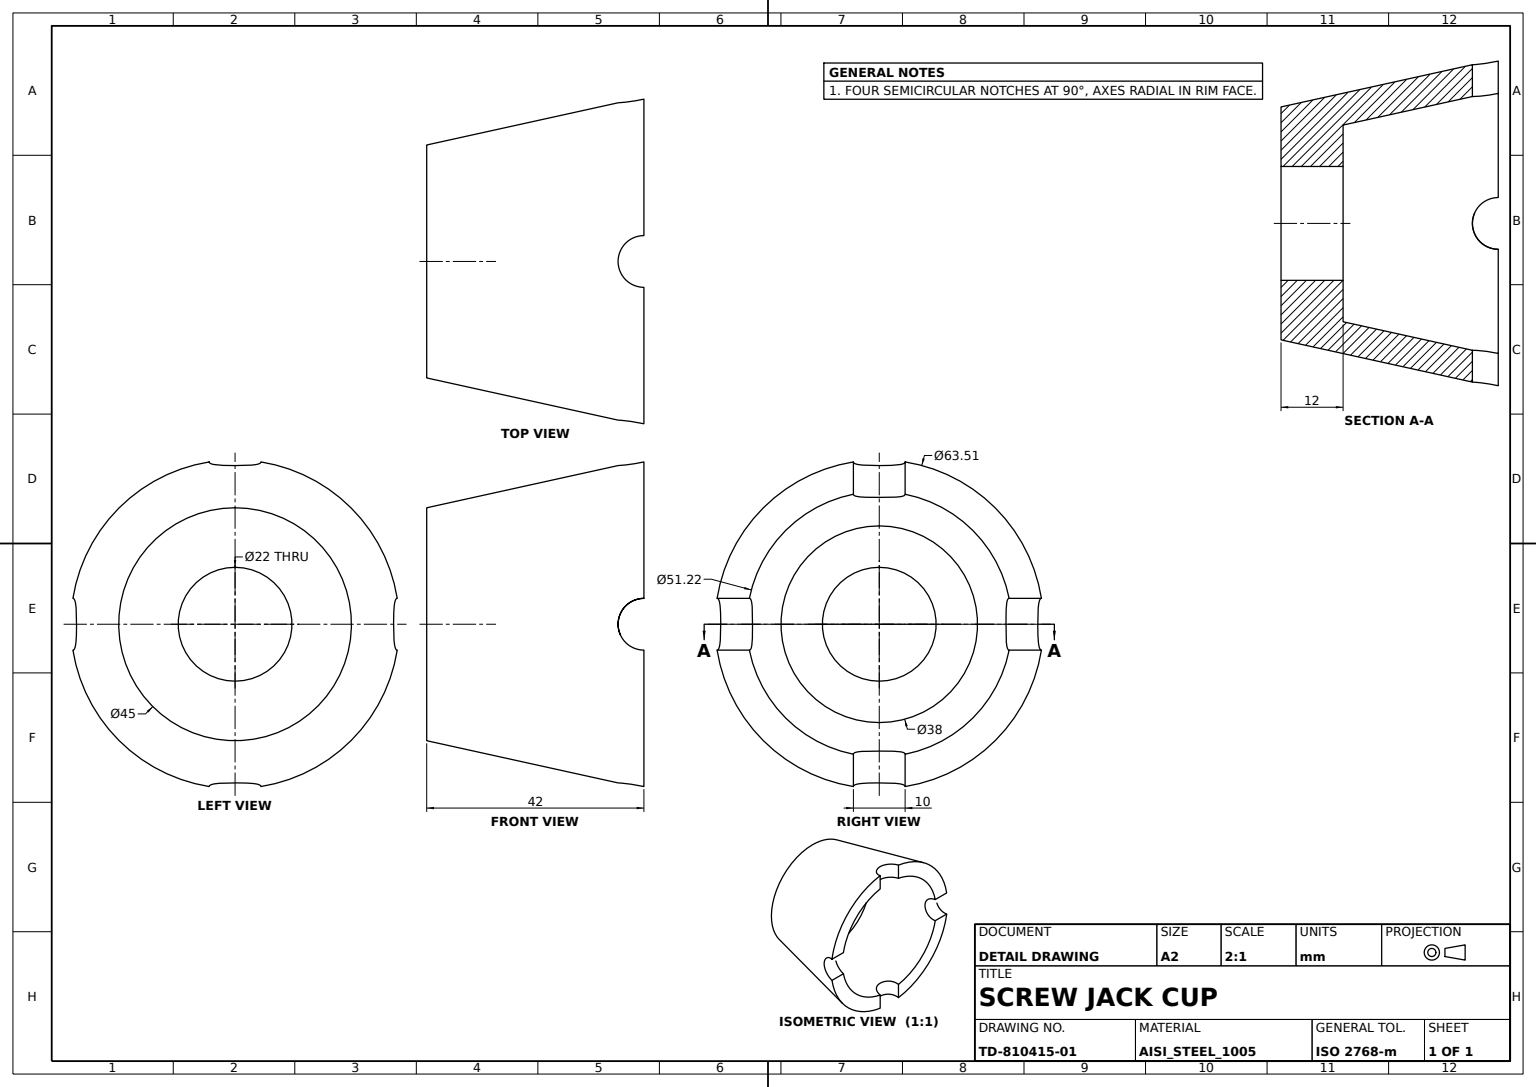
ISO-10303-21;
HEADER;
FILE_DESCRIPTION((''),'2;1');
FILE_NAME('','',(''),(''),'','','');
FILE_SCHEMA(('AUTOMOTIVE_DESIGN'));
ENDSEC;
DATA;
#1=APPLICATION_CONTEXT('');
#2=PRODUCT_CONTEXT('',#1,'mechanical');
#3=PRODUCT('','','',(#2));
#4=PRODUCT_DEFINITION_FORMATION('','',#3);
#5=PRODUCT_DEFINITION_CONTEXT('',#1,'design');
#6=PRODUCT_DEFINITION('','',#4,#5);
#7=PRODUCT_DEFINITION_SHAPE('','',#6);
#8=(LENGTH_UNIT()NAMED_UNIT(*)SI_UNIT(.MILLI.,.METRE.));
#9=(NAMED_UNIT(*)PLANE_ANGLE_UNIT()SI_UNIT($,.RADIAN.));
#10=(NAMED_UNIT(*)SI_UNIT($,.STERADIAN.)SOLID_ANGLE_UNIT());
#11=UNCERTAINTY_MEASURE_WITH_UNIT(LENGTH_MEASURE(0.005),#8,'distance_accuracy_value','');
#12=(GEOMETRIC_REPRESENTATION_CONTEXT(3)GLOBAL_UNCERTAINTY_ASSIGNED_CONTEXT((#11))GLOBAL_UNIT_ASSIGNED_CONTEXT((#8,#9,#10))REPRESENTATION_CONTEXT('',''));
#13=CARTESIAN_POINT('',(-42.,-25.116923,5.));
#14=VERTEX_POINT('',#13);
#15=CARTESIAN_POINT('',(-42.,-25.116923,-5.));
#16=VERTEX_POINT('',#15);
#17=CARTESIAN_POINT('',(-41.352204,-24.971396,5.));
#18=CARTESIAN_POINT('',(-40.063797,-24.73353,4.748155));
#19=CARTESIAN_POINT('',(-37.824304,-24.500184,3.278245));
#20=CARTESIAN_POINT('',(-36.450174,-24.515156,0.008023));
#21=CARTESIAN_POINT('',(-38.100183,-24.490988,-3.940384));
#22=CARTESIAN_POINT('',(-40.704221,-24.825828,-5.));
#23=B_SPLINE_CURVE_WITH_KNOTS('',3,(#13,#17,#18,#19,#20,#21,#22,#15),.UNSPECIFIED.,.F.,.F.,(4,1,1,1,1,4),(0.000000202,0.001964487,0.003928772,0.007857341,0.01178591,0.01571448),.UNSPECIFIED.);
#24=EDGE_CURVE('',#14,#16,#23,.T.);
#25=ORIENTED_EDGE('',*,*,#24,.T.);
#26=CARTESIAN_POINT('',(-42.,-31.357538,-5.));
#27=VERTEX_POINT('',#26);
#28=CARTESIAN_POINT('',(-42.,-40.,-5.));
#29=DIRECTION('',(0.,1.,0.));
#30=VECTOR('',#29,1000.);
#31=LINE('',#28,#30);
#32=EDGE_CURVE('',#27,#16,#31,.T.);
#33=ORIENTED_EDGE('',*,*,#32,.F.);
#34=CARTESIAN_POINT('',(-42.,-31.357538,5.));
#35=VERTEX_POINT('',#34);
#36=CARTESIAN_POINT('',(-41.351427,-31.212836,-5.));
#37=CARTESIAN_POINT('',(-40.064058,-30.966956,-4.747835));
#38=CARTESIAN_POINT('',(-37.826606,-30.682429,-3.280684));
#39=CARTESIAN_POINT('',(-36.448665,-30.633085,-0.008));
#40=CARTESIAN_POINT('',(-38.103157,-30.687587,3.942255));
#41=CARTESIAN_POINT('',(-40.702699,-31.068099,5.));
#42=B_SPLINE_CURVE_WITH_KNOTS('',3,(#26,#36,#37,#38,#39,#40,#41,#34),.UNSPECIFIED.,.F.,.F.,(4,1,1,1,1,4),(0.000000202,0.001966139,0.003932077,0.007863951,0.011795825,0.0157277),.UNSPECIFIED.);
#43=EDGE_CURVE('',#27,#35,#42,.T.);
#44=ORIENTED_EDGE('',*,*,#43,.T.);
#45=CARTESIAN_POINT('',(-42.,-40.,5.));
#46=LINE('',#45,#30);
#47=EDGE_CURVE('',#14,#35,#46,.F.);
#48=ORIENTED_EDGE('',*,*,#47,.F.);
#49=EDGE_LOOP('',(#25,#33,#44,#48));
#50=FACE_BOUND('',#49,.T.);
#51=CARTESIAN_POINT('',(-42.,-40.,0.));
#52=DIRECTION('',(0.,0.,1.));
#53=AXIS2_PLACEMENT_3D('',#51,#29,#52);
#54=CYLINDRICAL_SURFACE('',#53,5.);
#55=ADVANCED_FACE('',(#50),#54,.F.);
#56=CARTESIAN_POINT('',(-42.,5.,-31.357538));
#57=VERTEX_POINT('',#56);
#58=CARTESIAN_POINT('',(-42.,5.,-25.116923));
#59=VERTEX_POINT('',#58);
#60=CARTESIAN_POINT('',(-42.,5.,-40.));
#61=VECTOR('',#52,1000.);
#62=LINE('',#60,#61);
#63=EDGE_CURVE('',#57,#59,#62,.T.);
#64=ORIENTED_EDGE('',*,*,#63,.T.);
#65=CARTESIAN_POINT('',(-42.,25.116923,-5.));
#66=VERTEX_POINT('',#65);
#67=CARTESIAN_POINT('',(-42.,0.,0.));
#68=DIRECTION('',(-1.,0.,0.));
#69=AXIS2_PLACEMENT_3D('',#67,#68,#52);
#70=CIRCLE('',#69,25.60976);
#71=EDGE_CURVE('',#66,#59,#70,.T.);
#72=ORIENTED_EDGE('',*,*,#71,.F.);
#73=CARTESIAN_POINT('',(-42.,31.357538,-5.));
#74=VERTEX_POINT('',#73);
#75=CARTESIAN_POINT('',(-42.,40.,-5.));
#76=DIRECTION('',(0.,-1.,0.));
#77=VECTOR('',#76,1000.);
#78=LINE('',#75,#77);
#79=EDGE_CURVE('',#66,#74,#78,.F.);
#80=ORIENTED_EDGE('',*,*,#79,.T.);
#81=CIRCLE('',#69,31.753664);
#82=EDGE_CURVE('',#74,#57,#81,.T.);
#83=ORIENTED_EDGE('',*,*,#82,.T.);
#84=EDGE_LOOP('',(#64,#72,#80,#83));
#85=FACE_BOUND('',#84,.T.);
#86=CARTESIAN_POINT('',(-42.,31.753664,0.));
#87=DIRECTION('',(1.,0.,0.));
#88=DIRECTION('',(0.,0.,-1.));
#89=AXIS2_PLACEMENT_3D('',#86,#87,#88);
#90=PLANE('',#89);
#91=ADVANCED_FACE('',(#85),#90,.F.);
#92=CARTESIAN_POINT('',(0.,0.,22.5));
#93=VERTEX_POINT('',#92);
#94=CARTESIAN_POINT('',(0.,0.,0.));
#95=AXIS2_PLACEMENT_3D('',#94,#68,#52);
#96=CIRCLE('',#95,22.5);
#97=EDGE_CURVE('',#93,#93,#96,.T.);
#98=ORIENTED_EDGE('',*,*,#97,.T.);
#99=EDGE_LOOP('',(#98));
#100=FACE_BOUND('',#99,.T.);
#101=ORIENTED_EDGE('',*,*,#43,.F.);
#102=CARTESIAN_POINT('',(-42.,-5.,-31.357538));
#103=VERTEX_POINT('',#102);
#104=EDGE_CURVE('',#103,#27,#81,.T.);
#105=ORIENTED_EDGE('',*,*,#104,.F.);
#106=CARTESIAN_POINT('',(-41.351427,5.,-31.212836));
#107=CARTESIAN_POINT('',(-40.064058,4.747835,-30.966956));
#108=CARTESIAN_POINT('',(-37.826606,3.280684,-30.682429));
#109=CARTESIAN_POINT('',(-36.448665,0.008,-30.633085));
#110=CARTESIAN_POINT('',(-38.103157,-3.942255,-30.687587));
#111=CARTESIAN_POINT('',(-40.702699,-5.,-31.068099));
#112=B_SPLINE_CURVE_WITH_KNOTS('',3,(#56,#106,#107,#108,#109,#110,#111,#102),.UNSPECIFIED.,.F.,.F.,(4,1,1,1,1,4),(0.000000202,0.001966139,0.003932077,0.007863951,0.011795825,0.0157277),.UNSPECIFIED.);
#113=EDGE_CURVE('',#57,#103,#112,.T.);
#114=ORIENTED_EDGE('',*,*,#113,.F.);
#115=ORIENTED_EDGE('',*,*,#82,.F.);
#116=CARTESIAN_POINT('',(-42.,31.357538,5.));
#117=VERTEX_POINT('',#116);
#118=CARTESIAN_POINT('',(-41.351427,31.212836,5.));
#119=CARTESIAN_POINT('',(-40.064058,30.966956,4.747835));
#120=CARTESIAN_POINT('',(-37.826606,30.682429,3.280684));
#121=CARTESIAN_POINT('',(-36.448665,30.633085,0.008));
#122=CARTESIAN_POINT('',(-38.103157,30.687587,-3.942255));
#123=CARTESIAN_POINT('',(-40.702699,31.068099,-5.));
#124=B_SPLINE_CURVE_WITH_KNOTS('',3,(#116,#118,#119,#120,#121,#122,#123,#73),.UNSPECIFIED.,.F.,.F.,(4,1,1,1,1,4),(0.000000202,0.001966139,0.003932077,0.007863951,0.011795825,0.0157277),.UNSPECIFIED.);
#125=EDGE_CURVE('',#117,#74,#124,.T.);
#126=ORIENTED_EDGE('',*,*,#125,.F.);
#127=CARTESIAN_POINT('',(-42.,5.,31.357538));
#128=VERTEX_POINT('',#127);
#129=EDGE_CURVE('',#128,#117,#81,.T.);
#130=ORIENTED_EDGE('',*,*,#129,.F.);
#131=CARTESIAN_POINT('',(-42.,-5.,31.357538));
#132=VERTEX_POINT('',#131);
#133=CARTESIAN_POINT('',(-41.351427,-5.,31.212836));
#134=CARTESIAN_POINT('',(-40.064058,-4.747835,30.966956));
#135=CARTESIAN_POINT('',(-37.826606,-3.280684,30.682429));
#136=CARTESIAN_POINT('',(-36.448665,-0.008,30.633085));
#137=CARTESIAN_POINT('',(-38.103157,3.942255,30.687587));
#138=CARTESIAN_POINT('',(-40.702699,5.,31.068099));
#139=B_SPLINE_CURVE_WITH_KNOTS('',3,(#131,#133,#134,#135,#136,#137,#138,#127),.UNSPECIFIED.,.F.,.F.,(4,1,1,1,1,4),(0.000000202,0.001966139,0.003932077,0.007863951,0.011795825,0.0157277),.UNSPECIFIED.);
#140=EDGE_CURVE('',#132,#128,#139,.T.);
#141=ORIENTED_EDGE('',*,*,#140,.F.);
#142=EDGE_CURVE('',#35,#132,#81,.T.);
#143=ORIENTED_EDGE('',*,*,#142,.F.);
#144=EDGE_LOOP('',(#101,#105,#114,#115,#126,#130,#141,#143));
#145=FACE_BOUND('',#144,.T.);
#146=CONICAL_SURFACE('',#95,22.5,0.216860603);
#147=ADVANCED_FACE('',(#100,#145),#146,.T.);
#148=ORIENTED_EDGE('',*,*,#24,.F.);
#149=CARTESIAN_POINT('',(-42.,-5.,25.116923));
#150=VERTEX_POINT('',#149);
#151=EDGE_CURVE('',#14,#150,#70,.T.);
#152=ORIENTED_EDGE('',*,*,#151,.T.);
#153=CARTESIAN_POINT('',(-42.,5.,25.116923));
#154=VERTEX_POINT('',#153);
#155=CARTESIAN_POINT('',(-41.352204,5.,24.971396));
#156=CARTESIAN_POINT('',(-40.063797,4.748155,24.73353));
#157=CARTESIAN_POINT('',(-37.824304,3.278245,24.500184));
#158=CARTESIAN_POINT('',(-36.450174,0.008023,24.515156));
#159=CARTESIAN_POINT('',(-38.100183,-3.940384,24.490988));
#160=CARTESIAN_POINT('',(-40.704221,-5.,24.825828));
#161=B_SPLINE_CURVE_WITH_KNOTS('',3,(#153,#155,#156,#157,#158,#159,#160,#149),.UNSPECIFIED.,.F.,.F.,(4,1,1,1,1,4),(0.000000202,0.001964487,0.003928772,0.007857341,0.01178591,0.01571448),.UNSPECIFIED.);
#162=EDGE_CURVE('',#154,#150,#161,.T.);
#163=ORIENTED_EDGE('',*,*,#162,.F.);
#164=CARTESIAN_POINT('',(-42.,25.116923,5.));
#165=VERTEX_POINT('',#164);
#166=EDGE_CURVE('',#154,#165,#70,.T.);
#167=ORIENTED_EDGE('',*,*,#166,.T.);
#168=CARTESIAN_POINT('',(-41.352204,24.971396,-5.));
#169=CARTESIAN_POINT('',(-40.063797,24.73353,-4.748155));
#170=CARTESIAN_POINT('',(-37.824304,24.500184,-3.278245));
#171=CARTESIAN_POINT('',(-36.450174,24.515156,-0.008023));
#172=CARTESIAN_POINT('',(-38.100183,24.490988,3.940384));
#173=CARTESIAN_POINT('',(-40.704221,24.825828,5.));
#174=B_SPLINE_CURVE_WITH_KNOTS('',3,(#65,#168,#169,#170,#171,#172,#173,#164),.UNSPECIFIED.,.F.,.F.,(4,1,1,1,1,4),(0.000000202,0.001964487,0.003928772,0.007857341,0.01178591,0.01571448),.UNSPECIFIED.);
#175=EDGE_CURVE('',#66,#165,#174,.T.);
#176=ORIENTED_EDGE('',*,*,#175,.F.);
#177=ORIENTED_EDGE('',*,*,#71,.T.);
#178=CARTESIAN_POINT('',(-42.,-5.,-25.116923));
#179=VERTEX_POINT('',#178);
#180=CARTESIAN_POINT('',(-41.352204,-5.,-24.971396));
#181=CARTESIAN_POINT('',(-40.063797,-4.748155,-24.73353));
#182=CARTESIAN_POINT('',(-37.824304,-3.278245,-24.500184));
#183=CARTESIAN_POINT('',(-36.450174,-0.008023,-24.515156));
#184=CARTESIAN_POINT('',(-38.100183,3.940384,-24.490988));
#185=CARTESIAN_POINT('',(-40.704221,5.,-24.825828));
#186=B_SPLINE_CURVE_WITH_KNOTS('',3,(#178,#180,#181,#182,#183,#184,#185,#58),.UNSPECIFIED.,.F.,.F.,(4,1,1,1,1,4),(0.000000202,0.001964487,0.003928772,0.007857341,0.01178591,0.01571448),.UNSPECIFIED.);
#187=EDGE_CURVE('',#179,#59,#186,.T.);
#188=ORIENTED_EDGE('',*,*,#187,.F.);
#189=EDGE_CURVE('',#179,#16,#70,.T.);
#190=ORIENTED_EDGE('',*,*,#189,.T.);
#191=EDGE_LOOP('',(#148,#152,#163,#167,#176,#177,#188,#190));
#192=FACE_BOUND('',#191,.T.);
#193=CARTESIAN_POINT('',(-12.,0.,19.));
#194=VERTEX_POINT('',#193);
#195=CARTESIAN_POINT('',(-12.,0.,0.));
#196=AXIS2_PLACEMENT_3D('',#195,#68,#52);
#197=CIRCLE('',#196,19.);
#198=EDGE_CURVE('',#194,#194,#197,.T.);
#199=ORIENTED_EDGE('',*,*,#198,.F.);
#200=EDGE_LOOP('',(#199));
#201=FACE_BOUND('',#200,.T.);
#202=CONICAL_SURFACE('',#69,25.609760166,0.216860603);
#203=ADVANCED_FACE('',(#192,#201),#202,.F.);
#204=ORIENTED_EDGE('',*,*,#198,.T.);
#205=EDGE_LOOP('',(#204));
#206=FACE_BOUND('',#205,.T.);
#207=CARTESIAN_POINT('',(-12.,0.,11.));
#208=VERTEX_POINT('',#207);
#209=CIRCLE('',#196,11.);
#210=EDGE_CURVE('',#208,#208,#209,.T.);
#211=ORIENTED_EDGE('',*,*,#210,.F.);
#212=EDGE_LOOP('',(#211));
#213=FACE_BOUND('',#212,.T.);
#214=CARTESIAN_POINT('',(-12.,19.,0.));
#215=AXIS2_PLACEMENT_3D('',#214,#87,#88);
#216=PLANE('',#215);
#217=ADVANCED_FACE('',(#206,#213),#216,.F.);
#218=CARTESIAN_POINT('',(-42.,-5.,40.));
#219=VECTOR('',#88,1000.);
#220=LINE('',#218,#219);
#221=EDGE_CURVE('',#132,#150,#220,.T.);
#222=ORIENTED_EDGE('',*,*,#221,.T.);
#223=ORIENTED_EDGE('',*,*,#151,.F.);
#224=ORIENTED_EDGE('',*,*,#47,.T.);
#225=ORIENTED_EDGE('',*,*,#142,.T.);
#226=EDGE_LOOP('',(#222,#223,#224,#225));
#227=FACE_BOUND('',#226,.T.);
#228=ADVANCED_FACE('',(#227),#90,.F.);
#229=ORIENTED_EDGE('',*,*,#189,.F.);
#230=CARTESIAN_POINT('',(-42.,-5.,-40.));
#231=LINE('',#230,#61);
#232=EDGE_CURVE('',#179,#103,#231,.F.);
#233=ORIENTED_EDGE('',*,*,#232,.T.);
#234=ORIENTED_EDGE('',*,*,#104,.T.);
#235=ORIENTED_EDGE('',*,*,#32,.T.);
#236=EDGE_LOOP('',(#229,#233,#234,#235));
#237=FACE_BOUND('',#236,.T.);
#238=ADVANCED_FACE('',(#237),#90,.F.);
#239=CARTESIAN_POINT('',(-42.,40.,5.));
#240=LINE('',#239,#77);
#241=EDGE_CURVE('',#117,#165,#240,.T.);
#242=ORIENTED_EDGE('',*,*,#241,.T.);
#243=ORIENTED_EDGE('',*,*,#166,.F.);
#244=CARTESIAN_POINT('',(-42.,5.,40.));
#245=LINE('',#244,#219);
#246=EDGE_CURVE('',#154,#128,#245,.F.);
#247=ORIENTED_EDGE('',*,*,#246,.T.);
#248=ORIENTED_EDGE('',*,*,#129,.T.);
#249=EDGE_LOOP('',(#242,#243,#247,#248));
#250=FACE_BOUND('',#249,.T.);
#251=ADVANCED_FACE('',(#250),#90,.F.);
#252=ORIENTED_EDGE('',*,*,#113,.T.);
#253=ORIENTED_EDGE('',*,*,#232,.F.);
#254=ORIENTED_EDGE('',*,*,#187,.T.);
#255=ORIENTED_EDGE('',*,*,#63,.F.);
#256=EDGE_LOOP('',(#252,#253,#254,#255));
#257=FACE_BOUND('',#256,.T.);
#258=CARTESIAN_POINT('',(-42.,0.,-40.));
#259=AXIS2_PLACEMENT_3D('',#258,#52,#76);
#260=CYLINDRICAL_SURFACE('',#259,5.);
#261=ADVANCED_FACE('',(#257),#260,.F.);
#262=ORIENTED_EDGE('',*,*,#97,.F.);
#263=EDGE_LOOP('',(#262));
#264=FACE_BOUND('',#263,.T.);
#265=CARTESIAN_POINT('',(0.,0.,11.));
#266=VERTEX_POINT('',#265);
#267=CIRCLE('',#95,11.);
#268=EDGE_CURVE('',#266,#266,#267,.T.);
#269=ORIENTED_EDGE('',*,*,#268,.T.);
#270=EDGE_LOOP('',(#269));
#271=FACE_BOUND('',#270,.T.);
#272=CARTESIAN_POINT('',(0.,11.,0.));
#273=AXIS2_PLACEMENT_3D('',#272,#68,#52);
#274=PLANE('',#273);
#275=ADVANCED_FACE('',(#264,#271),#274,.F.);
#276=ORIENTED_EDGE('',*,*,#268,.F.);
#277=EDGE_LOOP('',(#276));
#278=FACE_BOUND('',#277,.T.);
#279=ORIENTED_EDGE('',*,*,#210,.T.);
#280=EDGE_LOOP('',(#279));
#281=FACE_BOUND('',#280,.T.);
#282=CYLINDRICAL_SURFACE('',#95,11.);
#283=ADVANCED_FACE('',(#278,#281),#282,.F.);
#284=ORIENTED_EDGE('',*,*,#125,.T.);
#285=ORIENTED_EDGE('',*,*,#79,.F.);
#286=ORIENTED_EDGE('',*,*,#175,.T.);
#287=ORIENTED_EDGE('',*,*,#241,.F.);
#288=EDGE_LOOP('',(#284,#285,#286,#287));
#289=FACE_BOUND('',#288,.T.);
#290=CARTESIAN_POINT('',(-42.,40.,0.));
#291=AXIS2_PLACEMENT_3D('',#290,#76,#88);
#292=CYLINDRICAL_SURFACE('',#291,5.);
#293=ADVANCED_FACE('',(#289),#292,.F.);
#294=ORIENTED_EDGE('',*,*,#140,.T.);
#295=ORIENTED_EDGE('',*,*,#246,.F.);
#296=ORIENTED_EDGE('',*,*,#162,.T.);
#297=ORIENTED_EDGE('',*,*,#221,.F.);
#298=EDGE_LOOP('',(#294,#295,#296,#297));
#299=FACE_BOUND('',#298,.T.);
#300=CARTESIAN_POINT('',(-42.,0.,40.));
#301=AXIS2_PLACEMENT_3D('',#300,#88,#68);
#302=CYLINDRICAL_SURFACE('',#301,5.);
#303=ADVANCED_FACE('',(#299),#302,.F.);
#304=CLOSED_SHELL('',(#55,#91,#147,#203,#217,#228,#238,#251,#261,#275,#283,#293,#303));
#305=MANIFOLD_SOLID_BREP('',#304);
#306=ADVANCED_BREP_SHAPE_REPRESENTATION('',(#305),#12);
#307=SHAPE_DEFINITION_REPRESENTATION(#7,#306);
ENDSEC;
END-ISO-10303-21;
